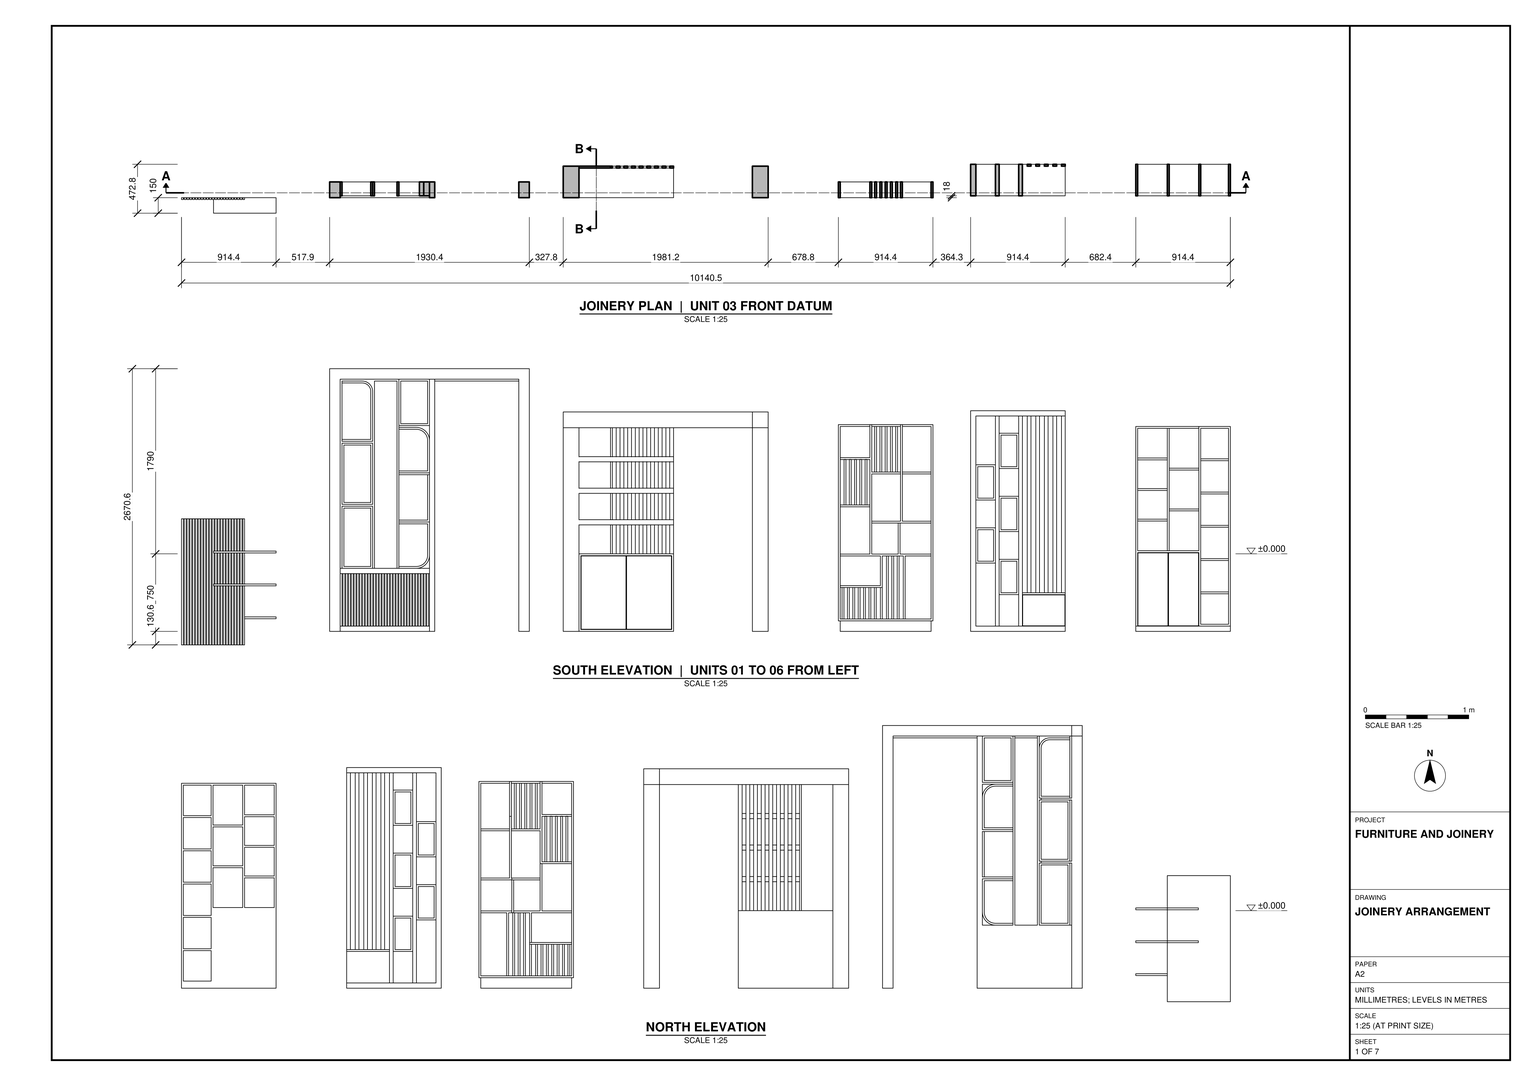
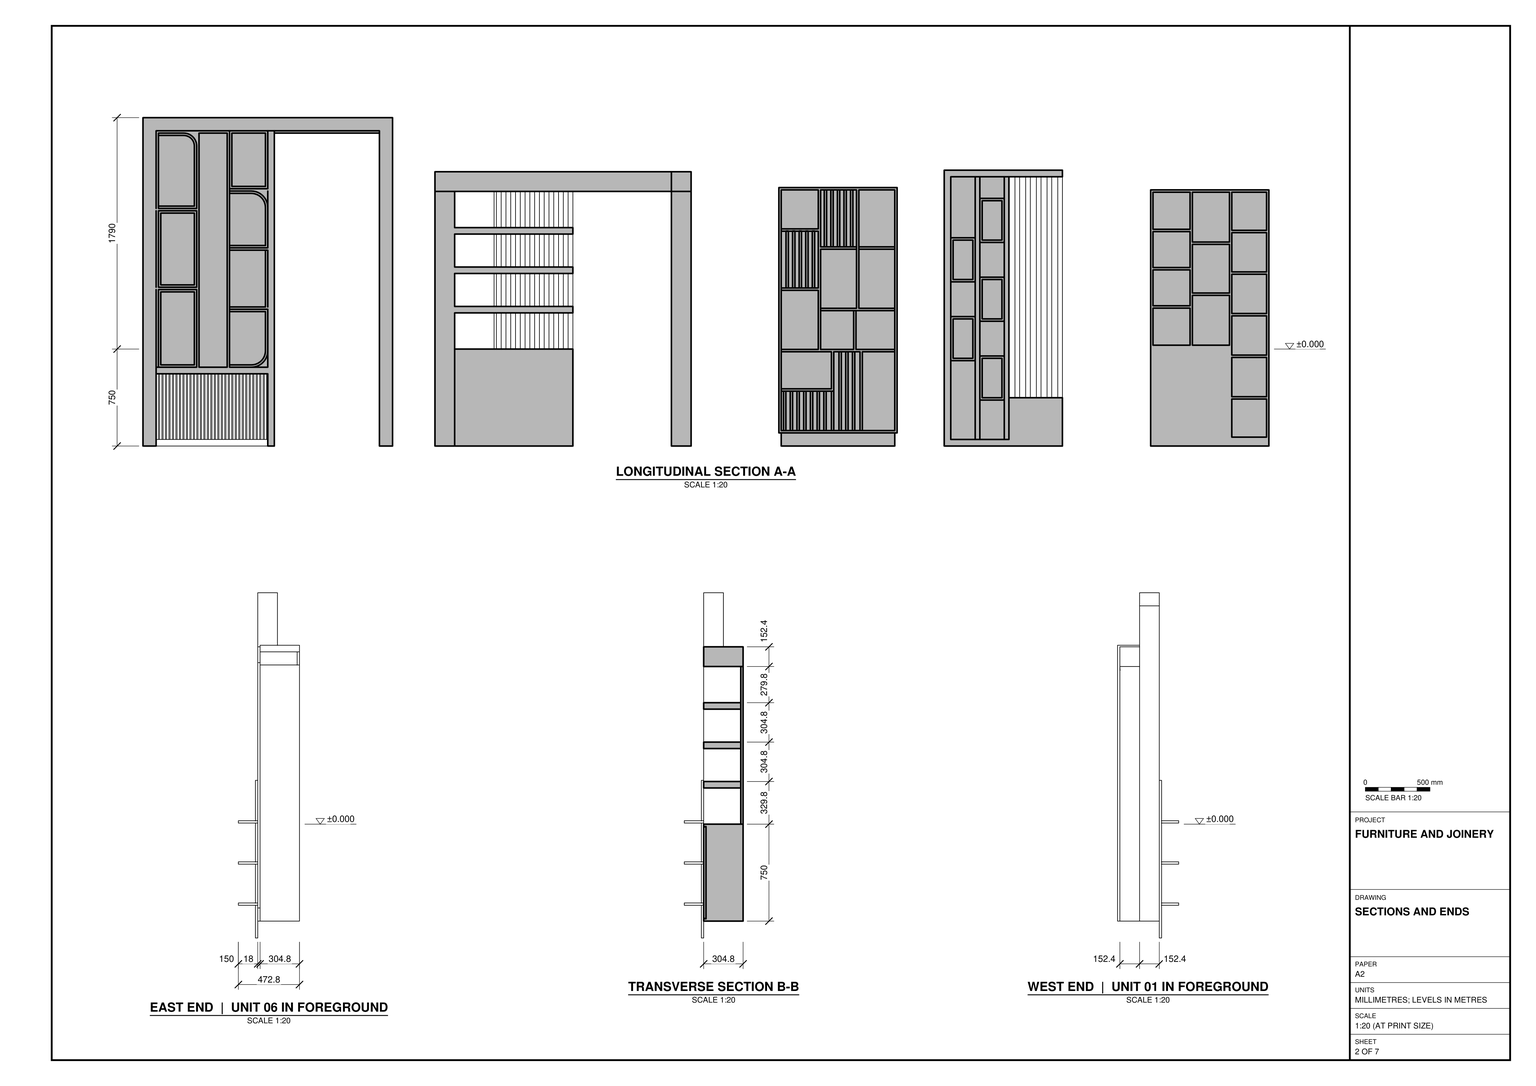
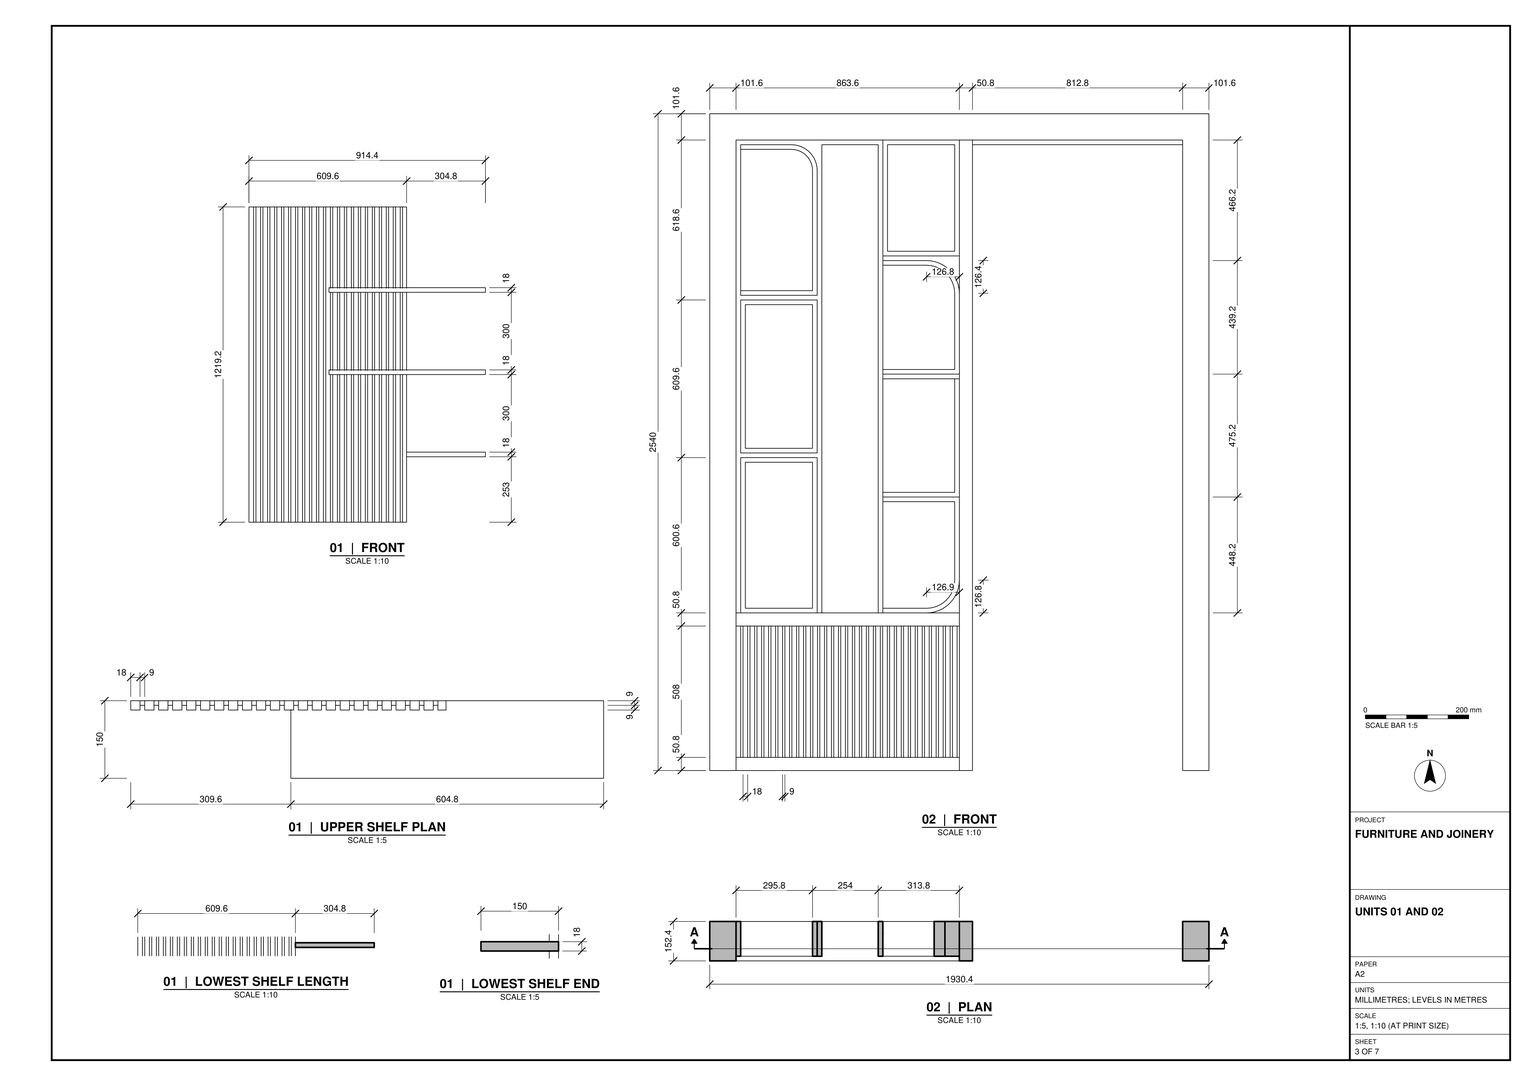
Build the six joinery units in SketchUp from task_files/diagram_01.pdf. Work in millimetres. The arrangement is 10140.5 mm long along X, 472.8 mm deep along Y and 2670.6 mm high along Z. Use the single reference level of 0 mm (±0.000 on the sheets). Set out the units from left to right as seen in the south elevation. Use the front of the third unit as the plan datum, and follow the drawn gaps, front-to-back offsets and base elevations.

Start with the low slatted panel and its three projecting shelves. Beside it, model the tall frame with rounded-corner compartments and a slatted lower panel on the left, leaving the bay on the right clear. The next frame has shelves over a two-panel base on the left and a clear opening on the right. For the remaining units, distinguish the staggered compartments with slatted infill, the narrow inset panels beside a tall slatted bay, and the three-column shelving layout. Use the plans and sections to give the frames, shelves, dividers and slats their drawn thicknesses and depths.

Keep each joinery unit in a separate group or component and use components for repeated parts such as identical slats. Any decor or loose items shown may be represented by suitable library components. Save one SketchUp model as output_files/six_display_and_shelving_units.skp.

# SketchUp Ruby script. Lengths in millimetres.
U = 1.mm
M = Sketchup.active_model
def pt(a) = Geom::Point3d.new(a.map { |v| v * U })
def face(e, loops, mat)
  f = e.add_face(loops[0].map { |a| pt(a) })
  loops[1..].each { |l| e.add_face(l.map { |a| pt(a) }).erase! }
  f.material = f.back_material = mat if mat
  f
end
# faces: each face lists its corners as indices into pts; further lists are holes
def faces(e, pts, list, mat = nil) = list.each { |f| face(e, (f[0].is_a?(Array) ? f : [f]).map { |l| l.map { |i| pts[i] } }, mat) }
# xy, xz, yz: faces in a plane at the given z, y or x. An outline is a flat list of corners, or four numbers for a rectangle; further outlines are holes
def ring(l) = l.size == 4 ? [[l[0], l[1]], [l[2], l[1]], [l[2], l[3]], [l[0], l[3]]] : l.each_slice(2).to_a
def flat(e, list, mat, &to3) = list.each { |f| face(e, (f[0].is_a?(Array) ? f : [f]).map { |l| ring(l).map { |u, v| to3.(u, v) } }, mat) }
def xy(e, z, list, mat = nil) = flat(e, list, mat) { |x, y| [x, y, z] }
def xz(e, y, list, mat = nil) = flat(e, list, mat) { |x, z| [x, y, z] }
def yz(e, x, list, mat = nil) = flat(e, list, mat) { |y, z| [x, y, z] }
def lines(e, pts, list) = list.each { |a, b| e.add_line(pt(pts[a]), pt(pts[b])) }
# prism: a flat outline (further loops are holes) pulled along v
def prism(e, loops, v, mat = nil)
  f = face(e, loops, mat); d = Geom::Vector3d.new(v.map { |x| x * U })
  f.pushpull(f.normal.samedirection?(d) ? d.length : -d.length)
end
def box(e, o, s, mat = nil) = prism(e, [[o, [o[0] + s[0], o[1], o[2]], [o[0] + s[0], o[1] + s[1], o[2]], [o[0], o[1] + s[1], o[2]]]], [0, 0, s[2]], mat)
def at(x, y, z, deg = 0) = Geom::Transformation.translation(pt([x, y, z])) * Geom::Transformation.rotation(ORIGIN, Z_AXIS, deg.degrees)
def axes(o, x, y, z) = Geom::Transformation.new([*x, 0, *y, 0, *z, 0, *pt(o).to_a, 1])
def part(name) = M.definitions.add(name)
# library, detail: a bought-in or finely detailed component or shape, given as its bounding box
def library(name, o, s) = part(name).tap { |d| box(d.entities, o, s) }
def detail(e, o, s) = box(e.add_group.entities, o, s)
def put(e, d, t, mat = nil) = e.add_instance(d, t).tap { |i| i.material = mat if mat }
def group(e, t, mat = nil) = e.add_group.tap { |g| g.transformation = t; g.material = mat if mat }.entities
root = M.entities
M.materials.add("[0046_Gold]").color = [249, 221, 90]
M.materials.add("[0082_LightSeaGreen]").color = [32, 178, 170]
M.materials.add("[0128_White]").color = [255, 255, 255]
M.materials.add("[Wood Bamboo]").color = [177, 105, 43]
M.materials.add("[Wood Cherry Original]").color = [152, 86, 42]
M.materials.add("[Wood Floor]").color = [155, 105, 61]
M.materials.add("[Wood Veneer 01]").color = [120, 70, 37]
c1 = library("Group\#1",[0,0,0],[609.6,18,1219.2])
c2 = library("Group\#4",[0,9,0],[864,18,508])
c3 = part("Group\#8")
box(c3.entities,[-2.6,0,0],[17.9,152.4,440.8])
c4 = part("Group\#10")
box(c4.entities,[0,0,0],[18,152.4,304.8])
c5 = part("Group\#9")
box(c5.entities,[0,0,0],[18,152.4,304.8])
c6 = part("Group\#16")
box(c6.entities,[0,0,0],[36,18,1709.2])
xy(root,0,[[0,132,18,150],[27,132,45,150],[54,132,72,150],[81,132,99,150],[108,132,126,150],
  [135,132,153,150],[162,132,180,150],[189,132,207,150],[216,132,234,150],[243,132,261,150],
  [270,132,288,150],[297,132,315,150],[324,132,342,150],[351,132,369,150],[378,132,396,150],
  [405,132,423,150],[432,132,450,150],[459,132,477,150],[486,132,504,150],[513,132,531,150],
  [540,132,558,150],[567,132,585,150],[594,132,609.6,150],[18,141,27,150],[45,141,54,150],
  [72,141,81,150],[99,141,108,150],[126,141,135,150],[153,141,162,150],[180,141,189,150],
  [207,141,216,150],[234,141,243,150],[261,141,270,150],[288,141,297,150],[315,141,324,150],
  [342,141,351,150],[369,141,378,150],[396,141,405,150],[423,141,432,150],[450,141,459,150],
  [477,141,486,150],[504,141,513,150],[531,141,540,150],[558,141,567,150],[585,141,594,150]],"[Wood Cherry Original]")
xy(root,130.6,[[1432.3,150,1533.9,302.4],[2397.5,150,2397.5,259,1533.9,259,1533.9,302.4,2448.3,302.4,2448.3,150],[3261.1,150,3362.7,302.4],[3690.6,150,3843,454.8],[3843,150,4757.4,454.8],
  [5519.4,150,5671.8,454.8],[7629.3,168,8543.7,472.8],[9226.1,168,10140.5,472.8]],"[Wood Cherry Original]")
xy(root,130.6,[[6368.6,168,7247,284.4]],"[Wood Veneer 01]")
xy(root,148.6,[[3861,150,4739.4,168]],"[Wood Cherry Original]")
xy(root,181.4,[[7869,168,7905,472.8],[8093.9,168,8129.9,472.8]])
xy(root,181.4,[[7680.1,168,7869,472.8],[7905,168,8093.9,472.8],[8129.9,168,8543.7,186],[9244.1,168,9835.7,186],[1533.9,259,2397.5,277]],"[Wood Cherry Original]")
xy(root,199.4,[[9853.7,168,10122.5,472.8]],"[Wood Cherry Original]")
xy(root,232.2,[[6368.6,168,7247,200],[6368.6,200,7247,284.4]])
xy(root,232.2,[[[6350.6,150,7265,302.4],[6368.6,168,7247,284.4]]],"[Wood Veneer 01]")
xy(root,250.2,[[6978.2,150,6996.2,302.4]])
xy(root,250.2,[[6368.6,150,6775,302.4],[6775,150,6978.2,302.4],[6996.2,150,7247,302.4]],"[Wood Veneer 01]")
xy(root,486.2,[[7905,168,8093.9,472.8]],"[0128_White]")
xy(root,486.2,[[8129.9,168,8543.7,186]],"[Wood Cherry Original]")
xy(root,494.1,[[9853.7,168,10122.5,472.8]],"[Wood Cherry Original]")
xy(root,504.2,[[7923,168,8075.9,472.8]])
xy(root,504.2,[[8129.9,168,8543.7,472.8]],"[Wood Cherry Original]")
xy(root,512.1,[[9853.7,168,10122.5,472.8]],"[Wood Cherry Original]")
xy(root,555,[[6368.6,150,6775,302.4]],"[Wood Veneer 01]")
xy(root,573,[[6368.6,150,6757,302.4]],"[Wood Veneer 01]")
xy(root,689.4,[[1533.9,150,2397.5,277]],"[Wood Cherry Original]")
xy(root,740.2,[[1533.9,150,2397.5,150,2397.5,168,2083.7,168,2083.7,302.4,1865.7,302.4,1865.7,168,1533.9,168],[1533.9,168,1551.9,302.4],[1551.9,168,1847.7,302.4],[2101.7,168,2270.5,302.4],[2270.5,168,2397.5,302.4]],"[Wood Cherry Original]")
xy(root,758.2,[[1569.9,168,1829.7,302.4],[2101.7,168,2270.5,302.4]],"[Wood Cherry Original]")
xy(root,791,[[7680.1,168,7869,472.8]],"[0128_White]")
xy(root,809,[[7698.1,168,7851,472.8],[7923,168,8075.9,472.8]],"[0128_White]")
xy(root,815.9,[[9853.7,168,10122.5,472.8]],"[Wood Cherry Original]")
xy(root,827,[[7905,168,8093.9,472.8]])
xy(root,833.9,[[9853.7,168,10122.5,472.8]],"[Wood Cherry Original]")
xy(root,859.8,[[6368.6,150,6757,302.4],[6775,150,6978.2,302.4],[6996.2,150,7247,302.4]],"[Wood Veneer 01]")
xy(root,862.6,[[3861,150,4739.4,168]],"[Wood Cherry Original]")
xy(root,877.8,[[6368.6,150,6655.4,302.4],[6673.4,150,6929,302.4],[6947,150,7247,302.4]],"[Wood Veneer 01]")
xy(root,880.6,[[3843,150,4757.4,454.8]],"[Wood Floor]")
xy(root,892.6,[[9244.1,168,9835.7,186]],"[Wood Cherry Original]")
xy(root,910.6,[[9244.1,168,9530.9,472.8],[9548.9,168,9835.7,472.8]],"[Wood Cherry Original]")
xy(root,1095.8,[[7905,168,8093.9,472.8]],"[0128_White]")
xy(root,1113.8,[[7698.1,168,7851,472.8],[7923,168,8075.9,472.8]],"[0128_White]")
xy(root,1131.8,[[7680.1,168,7869,472.8]],"[0128_White]")
xy(root,1137.6,[[9853.7,168,10122.5,472.8]],"[Wood Cherry Original]")
xy(root,1155.6,[[9853.7,168,10122.5,472.8]],"[Wood Cherry Original]")
xy(root,1160.4,[[3843,150,4757.4,436.8]],"[Wood Floor]")
xy(root,1170.4,[[2101.7,168,2379.5,302.4]],"[Wood Cherry Original]")
xy(root,1177.8,[[6929,150,6947,302.4]])
xy(root,1177.8,[[6673.4,150,6929,302.4],[6947,150,7247,302.4]],"[Wood Veneer 01]")
xy(root,1188.4,[[2101.7,168,2397.5,302.4]],"[Wood Cherry Original]")
xy(root,1195.8,[[6673.4,150,6951.2,302.4],[6969.2,150,7247,302.4]],"[Wood Veneer 01]")
xy(root,1197.4,[[9244.1,168,9530.9,472.8]],"[Wood Cherry Original]")
xy(root,1206.4,[[2101.7,168,2379.5,302.4]],"[Wood Cherry Original]")
xy(root,1210.4,[[3843,150,4757.4,436.8]],"[Wood Floor]")
xy(root,1215.4,[[9244.1,168,9530.9,472.8]],"[Wood Cherry Original]")
xy(root,1219.2,[[0,132,18,150]],"[Wood Cherry Original]")
xy(root,1296,[[9548.9,168,9835.7,472.8]],"[Wood Cherry Original]")
xy(root,1314,[[9548.9,168,9835.7,472.8]],"[Wood Cherry Original]")
xy(root,1322.8,[[1569.9,168,1829.7,302.4]],"[Wood Cherry Original]")
xy(root,1335,[[6368.6,150,6655.4,302.4]],"[Wood Veneer 01]")
xy(root,1340.8,[[1551.9,168,1829.7,302.4],[1829.7,168,1847.7,302.4]],"[Wood Cherry Original]")
xy(root,1353,[[6368.6,150,6655.4,302.4]],"[Wood Veneer 01]")
xy(root,1358.8,[[1551.9,168,1829.7,302.4],[1829.7,168,1847.7,302.4]],"[Wood Cherry Original]")
xy(root,1376.8,[[1569.9,168,1829.7,302.4]],"[Wood Cherry Original]")
xy(root,1400.6,[[7680.1,168,7869,472.8]],"[0128_White]")
xy(root,1418.6,[[7698.1,168,7851,472.8],[7923,168,8075.9,472.8]],"[0128_White]")
xy(root,1436.6,[[7905,168,8093.9,472.8]],"[0128_White]")
xy(root,1459.3,[[9853.7,168,10122.5,472.8]],"[Wood Cherry Original]")
xy(root,1465.2,[[3843,150,4757.4,436.8]],"[Wood Floor]")
xy(root,1477.3,[[9853.7,168,10122.5,472.8]],"[Wood Cherry Original]")
xy(root,1493.2,[[9244.1,168,9530.9,472.8]],"[Wood Cherry Original]")
xy(root,1511.2,[[9244.1,168,9530.9,472.8]],"[Wood Cherry Original]")
xy(root,1515.2,[[3843,150,4757.4,436.8]],"[Wood Floor]")
xy(root,1645.6,[[2101.7,168,2379.5,302.4],[2379.5,168,2397.5,302.4]],"[Wood Cherry Original]")
xy(root,1653,[[6673.4,150,6951.2,302.4],[6969.2,150,7247,302.4]],"[Wood Veneer 01]")
xy(root,1663.6,[[2101.7,168,2397.5,302.4]],"[Wood Cherry Original]")
xy(root,1671,[[6673.4,150,6951.2,302.4],[6969.2,150,7247,302.4]],"[Wood Veneer 01]")
xy(root,1681.6,[[2101.7,168,2379.5,302.4]],"[Wood Cherry Original]")
xy(root,1690.4,[[9548.9,168,9835.7,472.8]],"[Wood Cherry Original]")
xy(root,1705.4,[[7905,168,8093.9,472.8]],"[0128_White]")
xy(root,1708.4,[[9548.9,168,9835.7,472.8]],"[Wood Cherry Original]")
xy(root,1723.4,[[7698.1,168,7851,472.8],[7923,168,8075.9,472.8]],"[0128_White]")
xy(root,1741.4,[[7680.1,168,7869,472.8]],"[0128_White]")
xy(root,1770,[[3843,150,4757.4,436.8]],"[Wood Floor]")
xy(root,1781.1,[[9853.7,168,10122.5,472.8]],"[Wood Cherry Original]")
xy(root,1789,[[9244.1,168,9530.9,472.8]],"[Wood Cherry Original]")
xy(root,1792.2,[[6368.6,150,6655.4,302.4]],"[Wood Veneer 01]")
xy(root,1799.1,[[9853.7,168,10122.5,472.8]],"[Wood Cherry Original]")
xy(root,1807,[[9244.1,168,9530.9,472.8]],"[Wood Cherry Original]")
xy(root,1810.2,[[6368.6,150,6655.4,302.4]],"[Wood Veneer 01]")
xy(root,1820,[[3843,150,4757.4,436.8]],"[Wood Floor]")
xy(root,1932.4,[[1569.9,168,1829.7,302.4]],"[Wood Cherry Original]")
xy(root,1950.4,[[1551.9,168,1829.7,302.4],[1829.7,168,1847.7,302.4]],"[Wood Cherry Original]")
xy(root,1968.4,[[1551.9,168,1829.7,302.4],[1829.7,168,1847.7,302.4]],"[Wood Cherry Original]")
xy(root,1986.4,[[1551.9,168,1829.7,302.4]],"[Wood Cherry Original]")
xy(root,2028.2,[[7923,168,8075.9,472.8]],"[0128_White]")
xy(root,2046.2,[[7905,168,8093.9,472.8]],"[0128_White]")
xy(root,2084.8,[[2101.7,168,2269.9,302.4]],"[Wood Cherry Original]")
xy(root,2093.8,[[9244.1,168,9530.9,472.8],[9548.9,168,9835.7,472.8],[9853.7,168,10122.5,472.8]],"[Wood Cherry Original]")
xy(root,2099.8,[[3690.6,150,3843,454.8],[5519.4,150,5671.8,454.8]],"[Wood Cherry Original]")
xy(root,2099.8,[[3843,150,5519.4,454.8]],"[Wood Floor]")
xy(root,2102.8,[[2101.7,168,2270.5,302.4]],"[Wood Cherry Original]")
xy(root,2111.8,[[9226.1,168,10140.5,472.8]],"[Wood Cherry Original]")
xy(root,2111.8,[[6368.6,150,6655.4,302.4],[6673.4,150,6951.2,302.4],[6969.2,150,7247,302.4]],"[Wood Veneer 01]")
xy(root,2120.8,[[2101.7,168,2397.5,302.4]])
xy(root,2129.8,[[6350.6,150,7265,302.4]],"[Wood Veneer 01]")
xy(root,2138.8,[[2119.7,168,2379.5,302.4]],"[Wood Cherry Original]")
xy(root,2213.4,[[7869,168,7905,472.8],[8093.9,168,8129.9,472.8]])
xy(root,2213.4,[[7680.1,168,7869,472.8],[7905,168,8093.9,472.8],[8129.9,168,8543.7,472.8]],"[Wood Cherry Original]")
xy(root,2252.2,[[3690.6,150,5519.4,454.8],[5519.4,150,5671.8,454.8]],"[Wood Floor]")
xy(root,2264.2,[[7629.3,168,8543.7,472.8]],"[Wood Cherry Original]")
xy(root,2533,[[1551.9,168,1747.7,302.4]],"[Wood Cherry Original]")
xy(root,2551,[[1551.9,168,1747.7,302.4],[1865.7,168,2083.7,302.4],[2119.7,168,2379.5,302.4],[2448.3,168,3261.1,302.4]],"[Wood Cherry Original]")
xy(root,2569,[[1533.9,150,2397.5,168],[2397.5,150,2448.3,302.4],[2448.3,150,3261.1,168],[1533.9,168,1551.9,302.4],[1551.9,168,1847.7,302.4],
  [1847.7,168,1865.7,302.4],[1865.7,168,2083.7,302.4],[2083.7,168,2101.7,302.4],[2101.7,168,2397.5,302.4],[2448.3,168,3261.1,302.4]],"[Wood Cherry Original]")
xy(root,2670.6,[[1432.3,150,3362.7,302.4]],"[Wood Cherry Original]")
xz(root,150,[[1432.3,130.6,1533.9,130.6,1533.9,2569,3261.1,2569,3261.1,130.6,3362.7,130.6,3362.7,2670.6,1432.3,2670.6],[2397.5,130.6,2448.3,2569],[1533.9,689.4,2397.5,740.2]],"[Wood Cherry Original]")
xz(root,150,[[3690.6,130.6,3843,130.6,3843,1160.4,4757.4,1160.4,4757.4,1210.4,3843,1210.4,3843,1465.2,4757.4,1465.2,4757.4,1515.2,3843,1515.2,3843,1770,4757.4,1770,4757.4,1820,3843,1820,3843,2099.8,3690.6,2099.8],[[3843,130.6,4757.4,880.6],[3861,148.6,4739.4,862.6]],[5519.4,130.6,5671.8,2099.8],[3690.6,2099.8,5519.4,2252.2],[5519.4,2099.8,5671.8,2252.2]],"[Wood Floor]")
xz(root,150,[[6350.6,232.2,7265,232.2,7265,2129.8,6969.2,2129.8,6969.2,2111.8,7247,2111.8,7247,250.2,6368.6,250.2,6368.6,2111.8,6655.4,2111.8,6655.4,2129.8,6350.6,2129.8],[6978.2,250.2,6996.2,250.2,6996.2,859.8,7247,859.8,7247,877.8,6947,877.8,6947,1177.8,6929,1177.8,6929,877.8,6673.4,877.8,6673.4,1653,6951.2,1653,6951.2,1671,6673.4,1671,6673.4,2129.8,6655.4,2129.8,6655.4,1810.2,6368.6,1810.2,6368.6,1792.2,6655.4,1792.2,6655.4,877.8,6368.6,877.8,6368.6,859.8,6757,859.8,6757,573,6368.6,573,6368.6,555,6775,555,6775,859.8,6978.2,859.8],[6673.4,1177.8,7247,1177.8,7247,1195.8,6969.2,1195.8,6969.2,2129.8,6951.2,2129.8,6951.2,1195.8,6673.4,1195.8],[6368.6,1335,6655.4,1353],[6969.2,1653,7247,1671],
  [6673.4,2111.8,6951.2,2129.8]],"[Wood Veneer 01]")
xz(root,168,[[[1533.9,740.2,1551.9,740.2,1551.9,1340.8,1847.7,1340.8,1847.7,740.2,1865.7,740.2,1865.7,2551,2083.7,2551,2083.7,740.2,2101.7,740.2,2101.7,2569,1533.9,2569],[1551.9,1358.8,1847.7,1950.4],[1551.9,1968.4,1551.9,2551,1747.7,2551,1760.8,2550.1,1773.6,2547.6,1786,2543.4,1797.7,2537.6,1808.6,2530.3,1818.4,2521.7,1827.1,2511.9,1834.3,2501,1840.1,2489.3,1844.3,2476.9,1846.9,2464.1,1847.7,2451,1847.7,1968.4]],[[1551.9,740.2,1847.7,1340.8],[1569.9,758.2,1829.7,1322.8]],[2101.7,740.2,2270.5,740.2,2287.1,741.3,2303.4,744.5,2319.1,749.9,2334,757.2,2347.8,766.4,2360.3,777.4,2371.3,789.9,2380.5,803.7,2387.9,818.6,2393.2,834.3,2396.4,850.6,2397.5,867.2,2397.5,1188.4,2101.7,1188.4,2101.7,1170.4,2379.5,1170.4,2379.5,867.2,2378.6,853,2375.8,839,2371.2,825.5,2364.9,812.7,2357,800.9,2347.6,790.1,2336.9,780.7,2325,772.8,2312.2,766.5,2298.7,761.9,2284.8,759.1,2270.5,758.2,2101.7,758.2],[2101.7,1188.4,2397.5,1188.4,2397.5,1645.6,2379.5,1645.6,2379.5,1206.4,2101.7,1206.4],[[1551.9,1358.8,1847.7,1950.4],[1569.9,1376.8,1829.7,1932.4]],
  [2101.7,1645.6,2397.5,1663.6],[2101.7,1663.6,2397.5,1663.6,2397.5,1975.8,2396.4,1992.4,2393.2,2008.7,2387.9,2024.4,2380.5,2039.3,2371.3,2053.1,2360.3,2065.6,2347.8,2076.6,2334,2085.8,2319.1,2093.1,2317.2,2093.8,2303.4,2098.5,2287.1,2101.7,2270.5,2102.8,2101.7,2102.8,2101.7,2084.8,2269.9,2084.8,2284.7,2083.8,2298.7,2081.1,2311.4,2076.8,2312.2,2076.5,2325,2070.2,2336.9,2062.3,2347.6,2052.9,2357,2042.1,2364.9,2030.3,2371.2,2017.5,2375.8,2004,2378.6,1990,2379.5,1975.2,2379.5,1681.6,2101.7,1681.6],[1551.9,1968.4,1847.7,1968.4,1847.7,2451,1846.9,2464.1,1844.3,2476.9,1840.1,2489.3,1834.3,2501,1827.1,2511.9,1818.4,2521.7,1808.6,2530.3,1797.7,2537.6,1786,2543.4,1773.6,2547.6,1760.8,2550.1,1747.7,2551,1551.9,2551,1551.9,2533,1747.7,2533,1758.4,2532.3,1768.9,2530.2,1779.1,2526.8,1788.7,2522,1797.6,2516.1,1805.7,2509,1812.8,2500.9,1818.7,2492,1823.5,2482.4,1826.9,2472.2,1829,2461.7,1829.7,2451,1829.7,1986.4,1551.9,1986.4],[[2101.7,2120.8,2397.5,2569],[2119.7,2138.8,2379.5,2551]]],"[0046_Gold]")
xz(root,168,[[[7905,486.2,8093.9,827],[7923,504.2,8075.9,809]],[[7680.1,791,7869,1131.8],[7698.1,809,7851,1113.8]],[[7905,1095.8,8093.9,1436.6],[7923,1113.8,8075.9,1418.6]],[[7680.1,1400.6,7869,1741.4],[7698.1,1418.6,7851,1723.4]],[[7905,1705.4,8093.9,2046.2],[7923,1723.4,8075.9,2028.2]]],"[0128_White]")
xz(root,168,[[7629.3,130.6,8543.7,130.6,8543.7,181.4,7680.1,181.4,7680.1,2213.4,8543.7,2213.4,8543.7,2264.2,7629.3,2264.2],[9226.1,130.6,10140.5,181.4],[3861,148.6,4739.4,862.6],[7869,181.4,7905,2213.4],[8093.9,181.4,8129.9,2213.4],
  [[9226.1,181.4,9244.1,181.4,9244.1,892.6,9835.7,892.6,9835.7,181.4,10140.5,181.4,10140.5,2111.8,9835.7,2111.8,9835.7,910.6,9244.1,910.6,9244.1,2093.8,9835.7,2093.8,9835.7,2111.8,9226.1,2111.8],[9853.7,199.4,10122.5,2093.8]],[8129.9,486.2,8543.7,504.2],[9853.7,494.1,10122.5,512.1],[2270.5,740.2,2397.5,740.2,2397.5,867.2,2396.4,850.6,2393.2,834.3,2387.9,818.6,2380.5,803.7,2371.3,789.9,2360.3,777.4,2347.8,766.4,2334,757.2,2319.1,749.9,2303.4,744.5,2287.1,741.3],[9853.7,815.9,10122.5,833.9],
  [9530.9,910.6,9548.9,2093.8],[9853.7,1137.6,10122.5,1155.6],[9244.1,1197.4,9530.9,1215.4],[9548.9,1296,9835.7,1314],[9853.7,1459.3,10122.5,1477.3],
  [9244.1,1493.2,9530.9,1511.2],[9548.9,1690.4,9835.7,1708.4],[9853.7,1781.1,10122.5,1799.1],[9244.1,1789,9530.9,1807],[2397.5,1975.8,2397.5,2120.8,2101.7,2120.8,2101.7,2102.8,2270.5,2102.8,2287.1,2101.7,2303.4,2098.5,2317.2,2093.8,2319.1,2093.1,2334,2085.8,2347.8,2076.6,2360.3,2065.6,2371.3,2053.1,2380.5,2039.3,2387.9,2024.4,2393.2,2008.7,2396.4,1992.4],
  [2448.3,2551,3261.1,2569]],"[Wood Cherry Original]")
xz(root,168,[[6368.6,130.6,7247,232.2]],"[Wood Veneer 01]")
xz(root,186,[[8129.9,181.4,8543.7,486.2],[9244.1,181.4,9835.7,892.6]],"[Wood Cherry Original]")
xz(root,259,[[1533.9,130.6,2397.5,181.4]],"[Wood Cherry Original]")
xz(root,277,[[1533.9,181.4,2397.5,689.4]],"[Wood Cherry Original]")
xz(root,284.4,[[6368.6,130.6,7247,232.2]],"[Wood Veneer 01]")
xz(root,302.4,[[1432.3,130.6,1432.3,2569,1533.9,2569,1533.9,1968.4,1829.7,1968.4,1829.7,1950.4,1533.9,1950.4,1533.9,1358.8,1829.7,1358.8,1829.7,1340.8,1533.9,1340.8,1533.9,130.6],[3261.1,130.6,3261.1,2569,1533.9,2569,1533.9,2670.6,3362.7,2670.6,3362.7,130.6],[[1533.9,130.6,1533.9,740.2,1847.7,740.2,1847.7,1340.8,1829.7,1340.8,1829.7,1358.8,1847.7,1358.8,1847.7,1950.4,1829.7,1950.4,1829.7,1968.4,1847.7,1968.4,1847.7,2569,1865.7,2569,1865.7,740.2,2083.7,740.2,2083.7,2569,2101.7,2569,2101.7,2120.8,2397.5,2120.8,2397.5,2569,2448.3,2569,2448.3,130.6],[2101.7,740.2,2397.5,1188.4],[2101.7,1663.6,2397.5,2102.8],[2101.7,1206.4,2397.5,1645.6]],[1533.9,740.2,1551.9,1340.8],[[1551.9,740.2,1847.7,1340.8],[1569.9,758.2,1829.7,1322.8]],
  [2101.7,740.2,2101.7,758.2,2270.5,758.2,2284.8,759.1,2298.7,761.9,2312.2,766.5,2325,772.8,2336.9,780.7,2347.6,790.1,2357,800.9,2364.9,812.7,2371.2,825.5,2375.8,839,2378.6,853,2379.5,867.2,2379.5,1170.4,2101.7,1170.4,2101.7,1188.4,2397.5,1188.4,2397.5,867.2,2396.4,850.6,2393.2,834.3,2387.9,818.6,2380.5,803.7,2371.3,789.9,2360.3,777.4,2347.8,766.4,2334,757.2,2319.1,749.9,2303.4,744.5,2287.1,741.3,2270.5,740.2],[2270.5,740.2,2287.1,741.3,2303.4,744.5,2319.1,749.9,2334,757.2,2347.8,766.4,2360.3,777.4,2371.3,789.9,2380.5,803.7,2387.9,818.6,2393.2,834.3,2396.4,850.6,2397.5,867.2,2397.5,740.2],[2379.5,1206.4,2397.5,1645.6],[1533.9,1358.8,1551.9,1950.4],[[1551.9,1358.8,1847.7,1950.4],[1569.9,1376.8,1829.7,1932.4]],
  [2101.7,1663.6,2101.7,1681.6,2379.5,1681.6,2379.5,1975.2,2378.6,1990,2375.8,2004,2371.2,2017.5,2364.9,2030.3,2357,2042.1,2347.6,2052.9,2336.9,2062.3,2325,2070.2,2312.2,2076.5,2311.4,2076.8,2298.7,2081.1,2284.7,2083.8,2269.9,2084.8,2101.7,2084.8,2101.7,2102.8,2270.5,2102.8,2287.1,2101.7,2303.4,2098.5,2317.2,2093.8,2319.1,2093.1,2334,2085.8,2347.8,2076.6,2360.3,2065.6,2371.3,2053.1,2380.5,2039.3,2387.9,2024.4,2393.2,2008.7,2396.4,1992.4,2397.5,1975.8,2397.5,1663.6],[1533.9,1968.4,1551.9,2569],[1551.9,1968.4,1551.9,1986.4,1829.7,1986.4,1829.7,2451,1829,2461.7,1826.9,2472.2,1823.5,2482.4,1818.7,2492,1812.8,2500.9,1805.7,2509,1797.6,2516.1,1788.7,2522,1779.1,2526.8,1768.9,2530.2,1758.4,2532.3,1747.7,2533,1551.9,2533,1551.9,2551,1747.7,2551,1760.8,2550.1,1773.6,2547.6,1786,2543.4,1797.7,2537.6,1808.6,2530.3,1818.4,2521.7,1827.1,2511.9,1834.3,2501,1840.1,2489.3,1844.3,2476.9,1846.9,2464.1,1847.7,2451,1847.7,1968.4],[2397.5,1975.8,2396.4,1992.4,2393.2,2008.7,2387.9,2024.4,2380.5,2039.3,2371.3,2053.1,2360.3,2065.6,2347.8,2076.6,2334,2085.8,2319.1,2093.1,2317.2,2093.8,2303.4,2098.5,2287.1,2101.7,2270.5,2102.8,2397.5,2102.8],[[2101.7,2120.8,2397.5,2569],[2119.7,2138.8,2379.5,2551]],
  [1847.7,2451,1846.9,2464.1,1844.3,2476.9,1840.1,2489.3,1834.3,2501,1827.1,2511.9,1818.4,2521.7,1808.6,2530.3,1797.7,2537.6,1786,2543.4,1773.6,2547.6,1760.8,2550.1,1747.7,2551,1551.9,2551,1551.9,2569,1847.7,2569],[1865.7,2551,2083.7,2569],[2448.3,2551,3261.1,2569],[1432.3,2569,1533.9,2670.6]],"[Wood Cherry Original]")
xz(root,302.4,[[6350.6,232.2,6350.6,2129.8,6655.4,2129.8,6655.4,2111.8,6368.6,2111.8,6368.6,250.2,7247,250.2,7247,2111.8,6969.2,2111.8,6969.2,2129.8,7265,2129.8,7265,232.2],[6978.2,250.2,6978.2,859.8,6947,859.8,6947,877.8,7247,877.8,7247,859.8,6996.2,859.8,6996.2,250.2],[6368.6,555,6775,573],[6757,573,6757,859.8,6368.6,859.8,6368.6,877.8,6655.4,877.8,6655.4,1335,6673.4,1335,6673.4,877.8,6929,877.8,6929,859.8,6775,859.8,6775,573],[6929,859.8,6947,1177.8],
  [6673.4,1177.8,6947,1195.8],[6947,1177.8,6947,1195.8,6951.2,1195.8,6951.2,1792.2,6969.2,1792.2,6969.2,1195.8,7247,1195.8,7247,1177.8],[6368.6,1335,6368.6,1353,6655.4,1353,6655.4,1792.2,6368.6,1792.2,6368.6,1810.2,6655.4,1810.2,6655.4,2129.8,6673.4,2129.8,6673.4,1671,6951.2,1671,6951.2,1653,6673.4,1653,6673.4,1335],[6969.2,1653,7247,1671],[6951.2,1792.2,6969.2,2129.8],
  [6673.4,2111.8,6951.2,2129.8]],"[Wood Veneer 01]")
xz(root,436.8,[[3843,1160.4,4757.4,1210.4],[3843,1465.2,4757.4,1515.2],[3843,1770,4757.4,1820]],"[Wood Cherry Original]")
xz(root,454.8,[[3690.6,130.6,3843,2099.8],[3843,130.6,4757.4,880.6],[5519.4,130.6,5671.8,2099.8],[3690.6,2099.8,5519.4,2252.2],[5519.4,2099.8,5671.8,2252.2]],"[Wood Floor]")
xz(root,472.8,[[[7905,486.2,8093.9,827],[7923,504.2,8075.9,809]],[[7680.1,791,7869,1131.8],[7698.1,809,7851,1113.8]],[[7905,1095.8,8093.9,1436.6],[7923,1113.8,8075.9,1418.6]],[[7680.1,1400.6,7869,1741.4],[7698.1,1418.6,7851,1723.4]],[[7905,1705.4,8093.9,2046.2],[7923,1723.4,8075.9,2028.2]]],"[0128_White]")
xz(root,472.8,[[7629.3,130.6,7629.3,2264.2,8543.7,2264.2,8543.7,2213.4,7680.1,2213.4,7680.1,181.4,8543.7,181.4,8543.7,130.6],[[9226.1,130.6,10140.5,2111.8],[9548.9,1708.4,9835.7,2093.8],[9548.9,910.6,9835.7,1296],[9548.9,1314,9835.7,1690.4],[9244.1,910.6,9530.9,1197.4],[9244.1,1807,9530.9,2093.8],[9853.7,512.1,10122.5,815.9],[9853.7,833.9,10122.5,1137.6],[9853.7,1155.6,10122.5,1459.3],[9853.7,1477.3,10122.5,1781.1],[9244.1,1215.4,9530.9,1493.2],[9244.1,1511.2,9530.9,1789],[9853.7,199.4,10122.5,494.1],[9853.7,1799.1,10122.5,2093.8]],[7869,181.4,7905,2213.4],[8093.9,181.4,8129.9,2213.4],[8129.9,181.4,8543.7,486.2],
  [8129.9,486.2,8543.7,504.2]],"[Wood Cherry Original]")
yz(root,0,[[132,0,150,1219.2]],"[Wood Cherry Original]")
yz(root,1432.3,[[150,130.6,302.4,2569],[150,2569,302.4,2670.6]],"[Wood Cherry Original]")
yz(root,1533.9,[[150,130.6,259,130.6,259,181.4,277,181.4,277,689.4,150,689.4],[259,130.6,259,181.4,277,181.4,277,689.4,150,689.4,150,740.2,302.4,740.2,302.4,130.6],[150,740.2,168,1340.8],[168,740.2,302.4,1340.8],[150,1340.8,168,1358.8],
  [150,1358.8,168,1950.4],[168,1358.8,302.4,1950.4],[150,1950.4,168,1968.4],[150,1968.4,168,2569],[168,1968.4,302.4,2569]],"[Wood Cherry Original]")
yz(root,1551.9,[[168,740.2,302.4,1340.8],[168,1358.8,302.4,1950.4],[168,1968.4,302.4,1986.4],[168,1986.4,302.4,2533],[168,2533,302.4,2551]],"[Wood Cherry Original]")
yz(root,1569.9,[[168,758.2,302.4,1322.8],[168,1376.8,302.4,1932.4]],"[Wood Cherry Original]")
yz(root,1829.7,[[168,758.2,302.4,1322.8],[168,1376.8,302.4,1932.4],[168,1986.4,302.4,2451]],"[Wood Cherry Original]")
yz(root,1847.7,[[168,740.2,302.4,1340.8],[168,1358.8,302.4,1950.4],[168,1968.4,302.4,2451]],"[Wood Cherry Original]")
yz(root,1865.7,[[168,740.2,302.4,2551]],"[Wood Cherry Original]")
yz(root,2083.7,[[168,740.2,302.4,2551]],"[Wood Cherry Original]")
yz(root,2101.7,[[168,740.2,302.4,758.2],[168,758.2,302.4,1170.4],[168,1170.4,302.4,1188.4],[168,1188.4,302.4,1206.4],[168,1206.4,302.4,1645.6],
  [168,1645.6,302.4,1663.6],[168,1663.6,302.4,1681.6],[168,1681.6,302.4,2084.8],[168,2084.8,302.4,2102.8],[168,2102.8,302.4,2120.8],
  [168,2120.8,302.4,2569]],"[Wood Cherry Original]")
yz(root,2119.7,[[168,2138.8,302.4,2551]],"[Wood Cherry Original]")
yz(root,2379.5,[[168,867.2,302.4,1170.4],[168,1206.4,302.4,1645.6],[168,1681.6,302.4,1975.2],[168,2138.8,302.4,2551]],"[Wood Cherry Original]")
yz(root,2397.5,[[150,130.6,150,689.4,277,689.4,277,181.4,259,181.4,259,130.6],[150,740.2,168,2569],[168,740.2,302.4,867.2],[168,867.2,302.4,1188.4],[168,1206.4,302.4,1645.6],
  [168,1663.6,302.4,1975.8],[168,1975.8,302.4,2102.8],[168,2120.8,302.4,2569]],"[Wood Cherry Original]")
yz(root,2448.3,[[150,130.6,302.4,2551],[150,2551,168,2569],[168,2551,302.4,2569]],"[Wood Cherry Original]")
yz(root,3261.1,[[150,130.6,150,2569,168,2569,168,2551,302.4,2551,302.4,130.6],[168,2551,302.4,2569]],"[Wood Cherry Original]")
yz(root,3362.7,[[150,130.6,302.4,2670.6]],"[Wood Cherry Original]")
yz(root,3690.6,[[150,130.6,454.8,2099.8],[150,2099.8,454.8,2252.2]],"[Wood Floor]")
yz(root,3843,[[150,130.6,454.8,880.6],[436.8,880.6,454.8,880.6,454.8,2099.8,436.8,1804],[436.8,1804,454.8,2099.8,436.8,2099.8]],"[Wood Cherry Original]")
yz(root,3843,[[150,880.6,436.8,1160.4],[150,1210.4,436.8,1465.2],[150,1515.2,436.8,1770],[150,1820,436.8,2099.8]],"[Wood Floor]")
yz(root,3861,[[150,148.6,168,862.6]],"[Wood Cherry Original]")
yz(root,4739.4,[[150,148.6,168,862.6]],"[Wood Cherry Original]")
yz(root,4757.4,[[150,130.6,454.8,880.6],[150,1160.4,436.8,1210.4],[150,1465.2,436.8,1515.2],[150,1770,436.8,1820]],"[Wood Floor]")
yz(root,5519.4,[[150,2099.8,454.8,2252.2]],"[Wood Cherry Original]")
yz(root,5519.4,[[150,130.6,454.8,2099.8]],"[Wood Floor]")
yz(root,5671.8,[[150,130.6,454.8,2099.8],[150,2099.8,454.8,2252.2]],"[Wood Floor]")
yz(root,6350.6,[[150,232.2,302.4,2129.8]],"[Wood Veneer 01]")
yz(root,6368.6,[[150,555,302.4,573],[150,859.8,302.4,877.8],[150,1335,302.4,1353],[150,1792.2,302.4,1810.2]])
yz(root,6368.6,[[168,130.6,284.4,232.2],[150,250.2,302.4,555],[150,573,302.4,859.8],[150,877.8,302.4,1335],[150,1353,302.4,1792.2],
  [150,1810.2,302.4,2111.8]],"[Wood Veneer 01]")
yz(root,6655.4,[[150,877.8,302.4,1335],[150,1353,302.4,1792.2],[150,1810.2,302.4,2111.8]],"[Wood Veneer 01]")
yz(root,6673.4,[[150,1177.8,302.4,1195.8]])
yz(root,6673.4,[[150,877.8,302.4,1177.8],[150,1195.8,302.4,1653],[150,1671,302.4,2111.8]],"[Wood Veneer 01]")
yz(root,6757,[[150,573,302.4,859.8]],"[Wood Veneer 01]")
yz(root,6775,[[150,555,302.4,859.8]],"[Wood Veneer 01]")
yz(root,6929,[[150,877.8,302.4,1177.8]],"[Wood Veneer 01]")
yz(root,6947,[[150,877.8,302.4,1177.8]],"[Wood Veneer 01]")
yz(root,6951.2,[[150,1653,302.4,1671]])
yz(root,6951.2,[[150,1195.8,302.4,1653],[150,1671,302.4,2111.8]],"[Wood Veneer 01]")
yz(root,6969.2,[[150,1653,302.4,1671]])
yz(root,6969.2,[[150,1195.8,302.4,1653],[150,1671,302.4,2111.8]],"[Wood Veneer 01]")
yz(root,6978.2,[[150,250.2,302.4,859.8]],"[Wood Veneer 01]")
yz(root,6996.2,[[150,250.2,302.4,859.8]],"[Wood Veneer 01]")
yz(root,7247,[[150,859.8,302.4,877.8],[150,1177.8,302.4,1195.8],[150,1653,302.4,1671]])
yz(root,7247,[[168,130.6,284.4,232.2],[150,250.2,302.4,859.8],[150,877.8,302.4,1177.8],[150,1195.8,302.4,1653],[150,1671,302.4,2111.8]],"[Wood Veneer 01]")
yz(root,7265,[[150,232.2,302.4,2129.8]],"[Wood Veneer 01]")
yz(root,7629.3,[[168,130.6,472.8,2264.2]],"[Wood Cherry Original]")
yz(root,7680.1,[[168,791,472.8,1131.8],[168,1400.6,472.8,1741.4]])
yz(root,7680.1,[[168,181.4,472.8,791],[168,1131.8,472.8,1400.6],[168,1741.4,472.8,2213.4]],"[Wood Cherry Original]")
yz(root,7698.1,[[168,809,472.8,1113.8],[168,1418.6,472.8,1723.4]],"[0128_White]")
yz(root,7851,[[168,809,472.8,1113.8],[168,1418.6,472.8,1723.4]],"[0128_White]")
yz(root,7869,[[168,791,472.8,1131.8],[168,1131.8,472.8,1400.6],[168,1400.6,472.8,1741.4]])
yz(root,7869,[[168,181.4,472.8,791],[168,1741.4,472.8,2213.4]],"[Wood Cherry Original]")
yz(root,7905,[[168,486.2,472.8,827],[168,1095.8,472.8,1436.6],[168,1705.4,472.8,2046.2]])
yz(root,7905,[[168,181.4,472.8,486.2],[168,827,472.8,1095.8],[168,1436.6,472.8,1705.4],[168,2046.2,472.8,2213.4]],"[Wood Cherry Original]")
yz(root,7923,[[168,504.2,472.8,809]])
yz(root,7923,[[168,1113.8,472.8,1418.6],[168,1723.4,472.8,2028.2]],"[0128_White]")
yz(root,8075.9,[[168,504.2,472.8,809],[168,1113.8,472.8,1418.6],[168,1723.4,472.8,2028.2]],"[0128_White]")
yz(root,8093.9,[[168,486.2,472.8,827],[168,1095.8,472.8,1436.6],[168,1705.4,472.8,2046.2]])
yz(root,8093.9,[[168,181.4,472.8,486.2],[168,827,472.8,1095.8],[168,1436.6,472.8,1705.4],[168,2046.2,472.8,2213.4]],"[Wood Cherry Original]")
yz(root,8129.9,[[186,181.4,472.8,486.2],[168,486.2,472.8,504.2]])
yz(root,8129.9,[[168,181.4,186,486.2],[168,504.2,472.8,2213.4]],"[Wood Cherry Original]")
yz(root,8543.7,[[168,130.6,472.8,181.4],[186,181.4,472.8,181.4,472.8,504.2,168,504.2,168,486.2,186,486.2],[168,2213.4,472.8,2264.2]],"[Wood Cherry Original]")
yz(root,9226.1,[[168,130.6,472.8,892.6],[168,892.6,472.8,2111.8]],"[Wood Cherry Original]")
yz(root,9244.1,[[168,181.4,186,892.6],[168,910.6,472.8,1197.4],[168,1215.4,472.8,1493.2],[168,1511.2,472.8,1789],[168,1807,472.8,2093.8]],"[Wood Cherry Original]")
yz(root,9530.9,[[168,910.6,472.8,1197.4],[168,1215.4,472.8,1493.2],[168,1511.2,472.8,1789],[168,1807,472.8,2093.8]],"[Wood Cherry Original]")
yz(root,9548.9,[[168,910.6,472.8,1296],[168,1314,472.8,1690.4],[168,1708.4,472.8,2093.8]],"[Wood Cherry Original]")
yz(root,9835.7,[[168,181.4,186,892.6],[168,910.6,472.8,1296],[168,1314,472.8,1690.4],[168,1708.4,472.8,2093.8]],"[Wood Cherry Original]")
yz(root,9853.7,[[168,199.4,472.8,494.1],[168,512.1,472.8,815.9],[168,833.9,472.8,892.6],[168,892.6,472.8,910.6],[168,910.6,472.8,1137.6],
  [168,1155.6,472.8,1296],[168,1296,472.8,1314],[168,1314,472.8,1459.3],[168,1477.3,472.8,1690.4],[168,1690.4,472.8,1708.4],
  [168,1708.4,472.8,1781.1],[168,1799.1,472.8,2093.8]],"[Wood Cherry Original]")
yz(root,10122.5,[[168,199.4,472.8,494.1],[168,512.1,472.8,815.9],[168,833.9,472.8,1137.6],[168,1155.6,472.8,1459.3],[168,1477.3,472.8,1781.1],
  [168,1799.1,472.8,2093.8]],"[Wood Cherry Original]")
yz(root,10140.5,[[168,130.6,472.8,2111.8]],"[Wood Cherry Original]")
p = [[2270.5,302.4,740.2],[2270.5,168,740.2],[2287.1,168,741.3],[2287.1,302.4,741.3],[2303.4,168,744.5],[2303.4,302.4,744.5],
  [2319.1,168,749.9],[2319.1,302.4,749.9],[2334,168,757.2],[2334,302.4,757.2],[2347.8,168,766.4],[2347.8,302.4,766.4],
  [2270.5,302.4,758.2],[2270.5,168,758.2],[2284.8,168,759.1],[2284.8,302.4,759.1],[2298.7,168,761.9],[2298.7,302.4,761.9],
  [2312.2,168,766.5],[2312.2,302.4,766.5],[2360.3,168,777.4],[2360.3,302.4,777.4],[2325,168,772.8],[2325,302.4,772.8],
  [2336.9,168,780.7],[2336.9,302.4,780.7],[2371.3,168,789.9],[2371.3,302.4,789.9],[2347.6,168,790.1],[2347.6,302.4,790.1],
  [2380.5,168,803.7],[2380.5,302.4,803.7],[2357,168,800.9],[2357,302.4,800.9],[2364.9,168,812.7],[2364.9,302.4,812.7],
  [2387.9,168,818.6],[2387.9,302.4,818.6],[2371.2,168,825.5],[2371.2,302.4,825.5],[2393.2,168,834.3],[2393.2,302.4,834.3],
  [2375.8,168,839],[2375.8,302.4,839],[2396.4,168,850.6],[2396.4,302.4,850.6],[2378.6,168,853],[2378.6,302.4,853],
  [2397.5,168,867.2],[2397.5,302.4,867.2],[2379.5,168,867.2],[2379.5,302.4,867.2],[2379.5,302.4,1975.2],[2379.5,168,1975.2],
  [2378.6,168,1990],[2378.6,302.4,1990],[2397.5,302.4,1975.8],[2397.5,168,1975.8],[2396.4,168,1992.4],[2396.4,302.4,1992.4],
  [2375.8,168,2004],[2375.8,302.4,2004],[2393.2,168,2008.7],[2393.2,302.4,2008.7],[2371.2,168,2017.5],[2371.2,302.4,2017.5],
  [2387.9,168,2024.4],[2387.9,302.4,2024.4],[2364.9,168,2030.3],[2364.9,302.4,2030.3],[2380.5,168,2039.3],[2380.5,302.4,2039.3],
  [2357,168,2042.1],[2357,302.4,2042.1],[2371.3,168,2053.1],[2371.3,302.4,2053.1],[2347.6,168,2052.9],[2347.6,302.4,2052.9],
  [2336.9,168,2062.3],[2336.9,302.4,2062.3],[2360.3,168,2065.6],[2360.3,302.4,2065.6],[2325,168,2070.2],[2325,302.4,2070.2],
  [2347.8,168,2076.6],[2347.8,302.4,2076.6],[2312.2,168,2076.5],[2312.2,302.4,2076.5],[2311.4,168,2076.8],[2311.4,302.4,2076.8],
  [2334,168,2085.8],[2334,302.4,2085.8],[2298.7,168,2081.1],[2298.7,302.4,2081.1],[2284.7,168,2083.8],[2284.7,302.4,2083.8],
  [2269.9,168,2084.8],[2269.9,302.4,2084.8],[2319.1,168,2093.1],[2319.1,302.4,2093.1],[2317.2,168,2093.8],[2317.2,302.4,2093.8],
  [2303.4,168,2098.5],[2303.4,302.4,2098.5],[2287.1,168,2101.7],[2287.1,302.4,2101.7],[2270.5,168,2102.8],[2270.5,302.4,2102.8],
  [1829.7,302.4,2451],[1829.7,168,2451],[1829,168,2461.7],[1829,302.4,2461.7],[1847.7,168,2451],[1847.7,302.4,2451],
  [1846.9,302.4,2464.1],[1846.9,168,2464.1],[1826.9,168,2472.2],[1826.9,302.4,2472.2],[1844.3,302.4,2476.9],[1844.3,168,2476.9],
  [1823.5,168,2482.4],[1823.5,302.4,2482.4],[1840.1,302.4,2489.3],[1840.1,168,2489.3],[1818.7,168,2492],[1818.7,302.4,2492],
  [1834.3,302.4,2501],[1834.3,168,2501],[1812.8,168,2500.9],[1812.8,302.4,2500.9],[1805.7,168,2509],[1805.7,302.4,2509],
  [1827.1,302.4,2511.9],[1827.1,168,2511.9],[1797.6,168,2516.1],[1797.6,302.4,2516.1],[1818.4,302.4,2521.7],[1818.4,168,2521.7],
  [1788.7,168,2522],[1788.7,302.4,2522],[1808.6,302.4,2530.3],[1808.6,168,2530.3],[1779.1,168,2526.8],[1779.1,302.4,2526.8],
  [1768.9,168,2530.2],[1768.9,302.4,2530.2],[1758.4,168,2532.3],[1758.4,302.4,2532.3],[1797.7,302.4,2537.6],[1797.7,168,2537.6],
  [1747.7,168,2533],[1747.7,302.4,2533],[1786,302.4,2543.4],[1786,168,2543.4],[1773.6,302.4,2547.6],[1773.6,168,2547.6],
  [1760.8,302.4,2550.1],[1760.8,168,2550.1],[1747.7,302.4,2551],[1747.7,168,2551]]
faces(root,p,[[0,1,2,3],[3,2,4,5],[5,4,6,7],[7,6,8,9],[9,8,10,11],[12,13,14,15],[15,14,16,17],[17,16,18,19],
  [11,10,20,21],[19,18,22,23],[23,22,24,25],[21,20,26,27],[25,24,28,29],[27,26,30,31],[29,28,32,33],[33,32,34,35],
  [31,30,36,37],[35,34,38,39],[37,36,40,41],[39,38,42,43],[41,40,44,45],[43,42,46,47],[45,44,48,49],[47,46,50,51],
  [52,53,54,55],[56,57,58,59],[55,54,60,61],[59,58,62,63],[61,60,64,65],[63,62,66,67],[65,64,68,69],[67,66,70,71],
  [69,68,72,73],[71,70,74,75],[73,72,76,77],[77,76,78,79],[75,74,80,81],[79,78,82,83],[81,80,84,85],[83,82,86,87],
  [87,86,88,89],[85,84,90,91],[89,88,92,93],[93,92,94,95],[95,94,96,97],[91,90,98,99],[99,98,100,101],[101,100,102,103],
  [103,102,104,105],[106,107,105,104],[108,109,110,111],[112,113,114,115],[111,110,116,117],[118,119,115,114],[117,116,120,121],[122,123,119,118],
  [121,120,124,125],[126,127,123,122],[125,124,128,129],[129,128,130,131],[132,133,127,126],[131,130,134,135],[136,137,133,132],[135,134,138,139],
  [140,141,137,136],[139,138,142,143],[143,142,144,145],[145,144,146,147],[148,149,141,140],[147,146,150,151],[152,153,149,148],[154,155,153,152],
  [156,157,155,154],[158,159,157,156]],"[Wood Cherry Original]")
put(root,c1,at(0,132,0),"[Wood Cherry Original]")
g1 = group(root,at(609.6,132,253),"[Wood Cherry Original]")
box(g1,[0,-132,0],[304.8,150,18])
g2 = group(root,at(609.6,132,571),"[Wood Cherry Original]")
box(g2,[-300,-132,0],[604.8,150,18])
g3 = group(root,at(609.6,132,889),"[Wood Cherry Original]")
box(g3,[-300,-132,0],[604.8,150,18])
put(root,c2,at(1533.9,250,181.4),"[Wood Cherry Original]")
g4 = group(root,at(3843,454.8,880.6),"[Wood Floor]")
box(g4,[877.4,-18,0],[37,18,1219.2])
box(g4,[359.8,-18,0],[37,18,1219.2])
box(g4,[433.7,-18,0],[37,18,1219.2])
box(g4,[507.7,-18,0],[37,18,1219.2])
box(g4,[581.6,-18,0],[37,18,1219.2])
box(g4,[655.6,-18,0],[37,18,1219.2])
box(g4,[729.5,-18,0],[37,18,1219.2])
box(g4,[803.5,-18,0],[37,18,1219.2])
xy(g4,0,[[0,-18,304.8,0],[304.8,-18,322.8,0]])
xy(g4,1219.2,[[0,-18,304.8,0],[304.8,-18,322.8,0]])
xz(g4,-18,[[0,0,304.8,1219.2],[304.8,0,322.8,1219.2]])
xz(g4,0,[[0,0,304.8,1219.2],[304.8,0,322.8,1219.2]])
yz(g4,0,[[-18,0,0,1219.2]])
yz(g4,304.8,[[-18,0,0,1219.2]])
yz(g4,322.8,[[-18,0,0,1219.2]])
p = [[322.8,0,0],[359.8,0,0],[877.4,0,1219.2],[840.4,0,1219.2],[803.5,0,1219.2],[766.5,0,1219.2],
  [729.5,0,1219.2],[692.5,0,1219.2],[655.6,0,1219.2],[618.6,0,1219.2],[581.6,0,1219.2],[544.7,0,1219.2],
  [507.7,0,1219.2],[470.7,0,1219.2],[433.7,0,1219.2],[396.8,0,1219.2],[359.8,0,1219.2],[322.8,0,1219.2],
  [396.8,0,0],[433.7,0,0],[470.7,0,0],[507.7,0,0],[544.7,0,0],[581.6,0,0],
  [618.6,0,0],[655.6,0,0],[692.6,0,0],[729.5,0,0],[766.5,0,0],[803.5,0,0],
  [840.5,0,0],[877.4,0,0]]
lines(g4,p,[[0,1],[2,3],[4,5],[6,7],[8,9],[10,11],[12,13],[14,15],[16,17],[18,19],[20,21],[22,23],
  [24,25],[26,27],[28,29],[30,31]])
g5 = group(root,at(3861,150,148.6),"[0082_LightSeaGreen]")
xy(g5,3,[[3,0,436.2,18],[442.2,0,875.4,18]])
xy(g5,711,[[3,0,436.2,18],[442.2,0,875.4,18]])
xz(g5,0,[[3,3,436.2,711],[442.2,3,875.4,711]])
xz(g5,18,[[[0,0,439.2,714],[3,3,436.2,711]],[[439.2,0,878.4,714],[442.2,3,875.4,711]]])
yz(g5,3,[[0,3,18,711]])
yz(g5,436.2,[[0,3,18,711]])
yz(g5,442.2,[[0,3,18,711]])
yz(g5,875.4,[[0,3,18,711]])
put(root,c3,axes([6624.4,150,1353],[-1,0,0],[0,1,0],[0,0,1]),"[Wood Veneer 01]")
g6 = group(root,at(6757,150,250.2),"[Wood Veneer 01]")
box(g6,[0,0,0],[18,152.4,304.8])
g7 = group(root,at(6919.6,150,250.2),"[Wood Veneer 01]")
box(g7,[0,0,0],[18,152.4,609.6])
g8 = group(root,at(6815.6,150,250.2),"[Wood Veneer 01]")
box(g8,[0,0,0],[18,152.4,609.6])
g9 = group(root,at(6867.6,150,250.2),"[Wood Veneer 01]")
box(g9,[0,0,0],[18,152.4,609.6])
put(root,c4,axes([6612.4,150,250.2],[-1,0,0],[0,1,0],[0,0,1]),"[Wood Veneer 01]")
g10 = group(root,at(6716.4,150,250.2),"[Wood Veneer 01]")
box(g10,[-18,0,0],[18,152.4,304.8])
put(root,c5,axes([6664.4,150,250.2],[-1,0,0],[0,1,0],[0,0,1]),"[Wood Veneer 01]")
put(root,c4,axes([6508.5,150,250.2],[-1,0,0],[0,1,0],[0,0,1]),"[Wood Veneer 01]")
put(root,c5,axes([6560.5,150,250.2],[-1,0,0],[0,1,0],[0,0,1]),"[Wood Veneer 01]")
put(root,c5,axes([6456.6,150,250.2],[-1,0,0],[0,1,0],[0,0,1]),"[Wood Veneer 01]")
put(root,c4,axes([6404.6,150,250.2],[-1,0,0],[0,1,0],[0,0,1]),"[Wood Veneer 01]")
put(root,c3,axes([6573.6,150,1353],[-1,0,0],[0,1,0],[0,0,1]),"[Wood Veneer 01]")
put(root,c3,axes([6522.8,150,1353],[-1,0,0],[0,1,0],[0,0,1]),"[Wood Veneer 01]")
put(root,c3,axes([6472,150,1353],[-1,0,0],[0,1,0],[0,0,1]),"[Wood Veneer 01]")
put(root,c3,axes([6421.2,150,1353],[-1,0,0],[0,1,0],[0,0,1]),"[Wood Veneer 01]")
put(root,c3,axes([6869.4,150,1671],[-1,0,0],[0,1,0],[0,0,1]),"[Wood Veneer 01]")
put(root,c3,axes([6818.6,150,1671],[-1,0,0],[0,1,0],[0,0,1]),"[Wood Veneer 01]")
put(root,c3,axes([6717,150,1671],[-1,0,0],[0,1,0],[0,0,1]),"[Wood Veneer 01]")
put(root,c3,axes([6767.8,150,1671],[-1,0,0],[0,1,0],[0,0,1]),"[Wood Veneer 01]")
put(root,c3,axes([6920.2,150,1671],[-1,0,0],[0,1,0],[0,0,1]),"[Wood Veneer 01]")
g11 = group(root,at(8129.9,168,181.4),"[Wood Cherry Original]")
xy(g11,3,[[3,0,410.8,18]])
xy(g11,301.8,[[3,0,410.8,18]])
xz(g11,0,[[3,3,410.8,301.8]])
xz(g11,18,[[[0,0,413.8,304.8],[3,3,410.8,301.8]]])
yz(g11,3,[[0,3,18,301.8]])
yz(g11,410.8,[[0,3,18,301.8]])
put(root,c6,at(8176.6,454.8,504.2),"[Wood Cherry Original]")
put(root,c6,at(8259.4,454.8,504.2),"[Wood Cherry Original]")
put(root,c6,at(8342.2,454.8,504.2),"[Wood Cherry Original]")
put(root,c6,at(8424.9,454.8,504.2),"[Wood Cherry Original]")
put(root,c6,at(8507.7,454.8,504.2),"[Wood Cherry Original]")
g12 = group(root,at(9244.1,168,181.4),"[Wood Bamboo]")
xy(g12,3,[[3,0,292.8,8],[298.8,0,588.6,8]])
xy(g12,708.2,[[3,0,292.8,8],[298.8,0,588.6,8]])
xz(g12,0,[[3,3,292.8,708.2],[298.8,3,588.6,708.2]])
xz(g12,8,[[[0,0,295.8,711.2],[3,3,292.8,708.2]],[[295.8,0,591.6,711.2],[298.8,3,588.6,708.2]]])
yz(g12,3,[[0,3,8,708.2]])
yz(g12,292.8,[[0,3,8,708.2]])
yz(g12,298.8,[[0,3,8,708.2]])
yz(g12,588.6,[[0,3,8,708.2]])
